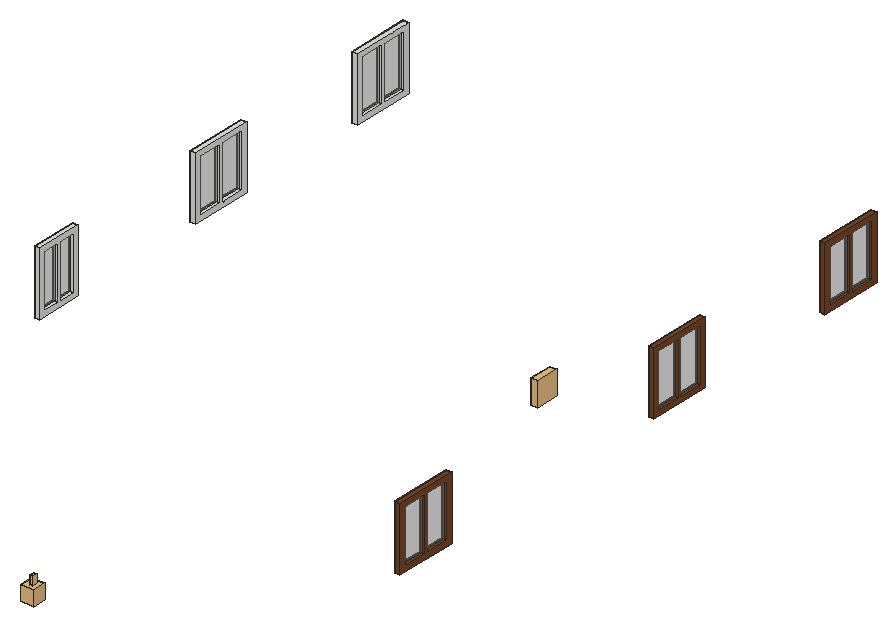
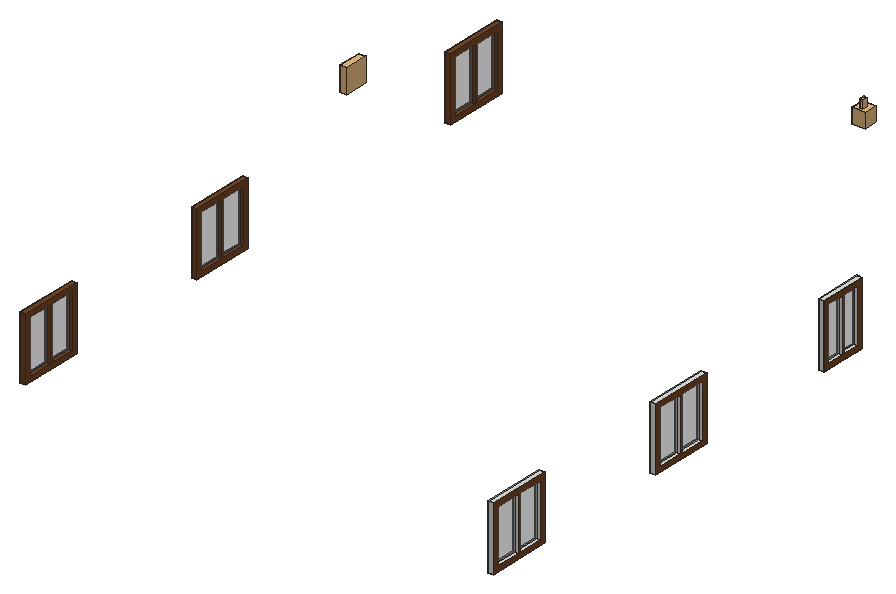
# SketchUp Ruby script. Lengths in inches.
U = 1.inch
M = Sketchup.active_model
def pt(a) = Geom::Point3d.new(a.map { |v| v * U })
def face(e, loops, mat)
  f = e.add_face(loops[0].map { |a| pt(a) })
  loops[1..].each { |l| e.add_face(l.map { |a| pt(a) }).erase! }
  f.material = f.back_material = mat if mat
  f
end
# faces: each face lists its corners as indices into pts; further lists are holes
def faces(e, pts, list, mat = nil) = list.each { |f| face(e, (f[0].is_a?(Array) ? f : [f]).map { |l| l.map { |i| pts[i] } }, mat) }
# xy, xz, yz: faces in a plane at the given z, y or x. An outline is a flat list of corners, or four numbers for a rectangle; further outlines are holes
def ring(l) = l.size == 4 ? [[l[0], l[1]], [l[2], l[1]], [l[2], l[3]], [l[0], l[3]]] : l.each_slice(2).to_a
def flat(e, list, mat, &to3) = list.each { |f| face(e, (f[0].is_a?(Array) ? f : [f]).map { |l| ring(l).map { |u, v| to3.(u, v) } }, mat) }
def xy(e, z, list, mat = nil) = flat(e, list, mat) { |x, y| [x, y, z] }
def xz(e, y, list, mat = nil) = flat(e, list, mat) { |x, z| [x, y, z] }
def yz(e, x, list, mat = nil) = flat(e, list, mat) { |y, z| [x, y, z] }
def lines(e, pts, list) = list.each { |a, b| e.add_line(pt(pts[a]), pt(pts[b])) }
# prism: a flat outline (further loops are holes) pulled along v
def prism(e, loops, v, mat = nil)
  f = face(e, loops, mat); d = Geom::Vector3d.new(v.map { |x| x * U })
  f.pushpull(f.normal.samedirection?(d) ? d.length : -d.length)
end
def box(e, o, s, mat = nil) = prism(e, [[o, [o[0] + s[0], o[1], o[2]], [o[0] + s[0], o[1] + s[1], o[2]], [o[0], o[1] + s[1], o[2]]]], [0, 0, s[2]], mat)
def at(x, y, z, deg = 0) = Geom::Transformation.translation(pt([x, y, z])) * Geom::Transformation.rotation(ORIGIN, Z_AXIS, deg.degrees)
def axes(o, x, y, z) = Geom::Transformation.new([*x, 0, *y, 0, *z, 0, *pt(o).to_a, 1])
def part(name) = M.definitions.add(name)
# library, detail: a bought-in or finely detailed component or shape, given as its bounding box
def library(name, o, s) = part(name).tap { |d| box(d.entities, o, s) }
def detail(e, o, s) = box(e.add_group.entities, o, s)
def put(e, d, t, mat = nil) = e.add_instance(d, t).tap { |i| i.material = mat if mat }
def group(e, t, mat = nil) = e.add_group.tap { |g| g.transformation = t; g.material = mat if mat }.entities
root = M.entities
M.materials.add("[Translucent Glass Gray]").color = [128, 128, 128]
M.materials["[Translucent Glass Gray]"].alpha = 0.5
M.materials.add("[Wood Veneer 01]").color = [120, 70, 37]
c1 = library("Spot Light\#1",[-5.1,-5.1,-11.05],[10.2,10.2,11.05])
c2 = library("[SKP_VZ_MOD_01]_WALL_LIGHT",[-1.1,-1.22,0],[3.54,2.36,6.3])
c3 = part("Group21\#2")
xy(c3.entities,0,[[-20.0625,-20.0625,-0.59,20.0625],[0.59,-20.0625,20.0625,20.0625]])
c4 = part("Group20\#3")
prism(c4.entities,[[[-24,24,0],[24,24,0],[24,-24,0],[-24,-24,0]],[[-20.0625,-20.0625,0],[-0.59,-20.0625,0],[-0.59,20.0625,0],[-20.0625,20.0625,0]],[[20.0625,20.0625,0],[0.59,20.0625,0],[0.59,-20.0625,0],[20.0625,-20.0625,0]]],[0,0,4],"[Wood Veneer 01]")
put(c4.entities,c3,at(0,0,2),"[Translucent Glass Gray]")
c5 = part("Group90\#1")
xy(c5.entities,0,[[-20.0625,-20.0625,-0.59,20.0625],[0.59,-20.0625,20.0625,20.0625]])
c6 = part("Group89\#1")
xy(c6.entities,0,[[[-24,-24,24,24],[-20.0625,-20.0625,-0.59,20.0625],[0.59,-20.0625,20.0625,20.0625]]])
xy(c6.entities,4,[[[-24,-24,24,24],[-20.0625,-20.0625,-0.59,20.0625],[0.59,-20.0625,20.0625,20.0625]]],"[Wood Veneer 01]")
xz(c6.entities,-24,[[-24,0,24,4]])
xz(c6.entities,-20.0625,[[-20.0625,0,-0.59,4],[0.59,0,20.0625,4]])
xz(c6.entities,20.0625,[[-20.0625,0,-0.59,4],[0.59,0,20.0625,4]])
xz(c6.entities,24,[[-24,0,24,4]])
yz(c6.entities,-24,[[-24,0,24,4]])
yz(c6.entities,-20.0625,[[-20.0625,0,20.0625,4]])
yz(c6.entities,-0.59,[[-20.0625,0,20.0625,4]])
yz(c6.entities,0.59,[[-20.0625,0,20.0625,4]])
yz(c6.entities,20.0625,[[-20.0625,0,20.0625,4]])
yz(c6.entities,24,[[-24,0,24,4]])
put(c6.entities,c5,at(0,0,2),"[Translucent Glass Gray]")
c7 = part("Group94\#1")
xy(c7.entities,0,[[-14.01,-20.0625,-0.59,20.0625],[0.59,-20.0625,14.01,20.0625]])
c8 = part("Group93\#1")
xy(c8.entities,0,[[[-17.94,-24,17.94,24],[0.59,-20.0625,14.01,20.0625],[-14.01,-20.0625,-0.59,20.0625]]])
xy(c8.entities,4,[[[-17.94,-24,17.94,24],[0.59,-20.0625,14.01,20.0625],[-14.01,-20.0625,-0.59,20.0625]]],"[Wood Veneer 01]")
xz(c8.entities,-24,[[-17.94,0,17.94,4]])
xz(c8.entities,-20.0625,[[-14.01,0,-0.59,4],[0.59,0,14.01,4]])
xz(c8.entities,20.0625,[[-14.01,0,-0.59,4],[0.59,0,14.01,4]])
xz(c8.entities,24,[[-17.94,0,17.94,4]])
yz(c8.entities,-17.94,[[-24,0,24,4]])
yz(c8.entities,-14.01,[[-20.0625,0,20.0625,4]])
yz(c8.entities,-0.59,[[-20.0625,0,20.0625,4]])
yz(c8.entities,0.59,[[-20.0625,0,20.0625,4]])
yz(c8.entities,14.01,[[-20.0625,0,20.0625,4]])
yz(c8.entities,17.94,[[-24,0,24,4]])
put(c8.entities,c7,at(0,0,2),"[Translucent Glass Gray]")
c9 = library("Agrupar\#12",[-0.01,0,0],[12.55,78.74,39.39])
p = [[0,283.65,84],[0,319.54,84],[0,319.54,36],[0,283.65,36]]
lines(root,p,[[0,1],[1,2],[2,3],[3,0]])
put(root,c1,at(189.4,45.0625,27.84))
put(root,c2,at(189.4,45.3,27.54,90))
put(root,c4,axes([356.05,201.2,60],[0,1,0],[0,0,1],[1,0,0]))
put(root,c4,axes([356.05,439.46,60],[0,1,0],[0,0,1],[1,0,0]))
put(root,c4,axes([356.05,600.375,60],[0,1,0],[0,0,1],[1,0,0]))
put(root,c6,axes([4,605.94,60],[0,-1,0],[0,0,1],[-1,0,0]))
put(root,c6,axes([4,453.75,60],[0,-1,0],[0,0,1],[-1,0,0]))
put(root,c8,axes([4,301.6,60],[0,-1,0],[0,0,1],[-1,0,0]))
put(root,c9,axes([364.97,318.42,96],[-0.45,0,0],[0,-0.2286,0],[0,0,0.45697]))
